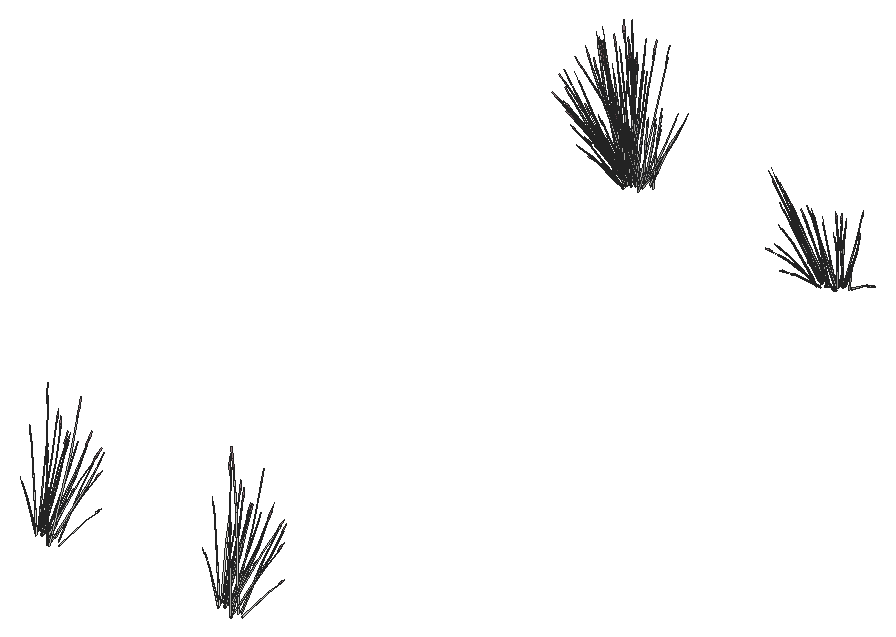
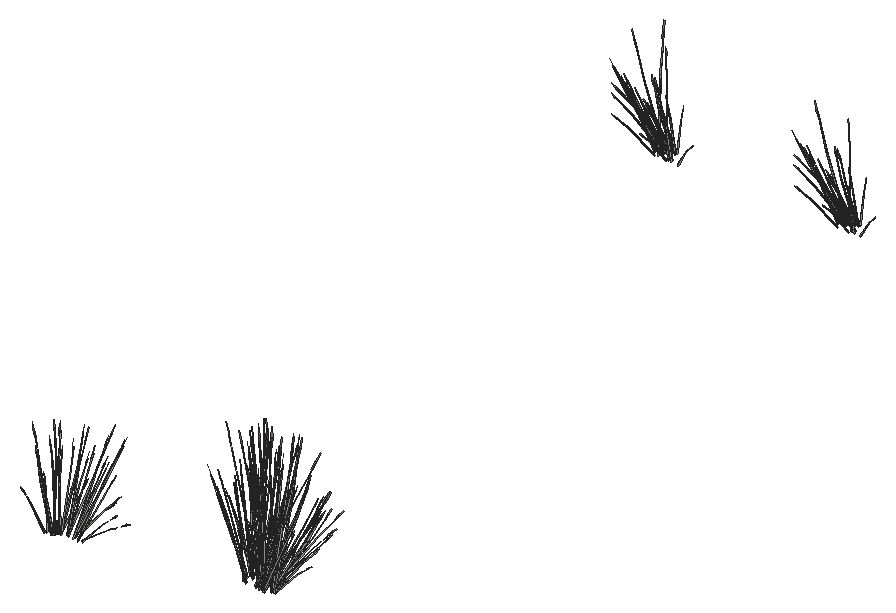
# SketchUp Ruby script. Lengths in millimetres.
U = 1.mm
M = Sketchup.active_model
def pt(a) = Geom::Point3d.new(a.map { |v| v * U })
def face(e, loops, mat)
  f = e.add_face(loops[0].map { |a| pt(a) })
  loops[1..].each { |l| e.add_face(l.map { |a| pt(a) }).erase! }
  f.material = f.back_material = mat if mat
  f
end
# faces: each face lists its corners as indices into pts; further lists are holes
def faces(e, pts, list, mat = nil) = list.each { |f| face(e, (f[0].is_a?(Array) ? f : [f]).map { |l| l.map { |i| pts[i] } }, mat) }
# xy, xz, yz: faces in a plane at the given z, y or x. An outline is a flat list of corners, or four numbers for a rectangle; further outlines are holes
def ring(l) = l.size == 4 ? [[l[0], l[1]], [l[2], l[1]], [l[2], l[3]], [l[0], l[3]]] : l.each_slice(2).to_a
def flat(e, list, mat, &to3) = list.each { |f| face(e, (f[0].is_a?(Array) ? f : [f]).map { |l| ring(l).map { |u, v| to3.(u, v) } }, mat) }
def xy(e, z, list, mat = nil) = flat(e, list, mat) { |x, y| [x, y, z] }
def xz(e, y, list, mat = nil) = flat(e, list, mat) { |x, z| [x, y, z] }
def yz(e, x, list, mat = nil) = flat(e, list, mat) { |y, z| [x, y, z] }
def lines(e, pts, list) = list.each { |a, b| e.add_line(pt(pts[a]), pt(pts[b])) }
# prism: a flat outline (further loops are holes) pulled along v
def prism(e, loops, v, mat = nil)
  f = face(e, loops, mat); d = Geom::Vector3d.new(v.map { |x| x * U })
  f.pushpull(f.normal.samedirection?(d) ? d.length : -d.length)
end
def box(e, o, s, mat = nil) = prism(e, [[o, [o[0] + s[0], o[1], o[2]], [o[0] + s[0], o[1] + s[1], o[2]], [o[0], o[1] + s[1], o[2]]]], [0, 0, s[2]], mat)
def at(x, y, z, deg = 0) = Geom::Transformation.translation(pt([x, y, z])) * Geom::Transformation.rotation(ORIGIN, Z_AXIS, deg.degrees)
def axes(o, x, y, z) = Geom::Transformation.new([*x, 0, *y, 0, *z, 0, *pt(o).to_a, 1])
def part(name) = M.definitions.add(name)
# library, detail: a bought-in or finely detailed component or shape, given as its bounding box
def library(name, o, s) = part(name).tap { |d| box(d.entities, o, s) }
def detail(e, o, s) = box(e.add_group.entities, o, s)
def put(e, d, t, mat = nil) = e.add_instance(d, t).tap { |i| i.material = mat if mat }
def group(e, t, mat = nil) = e.add_group.tap { |g| g.transformation = t; g.material = mat if mat }.entities
root = M.entities
M.materials.add("LightPink_Translucent").color = [144, 107, 117]
M.materials["LightPink_Translucent"].alpha = 0.8
c1 = part("blade")
p = [[54.7,5.3,558.8],[0,4.4,0],[2.3,11.5,0],[55.5,7.8,558.8],[58.2,7.8,558.8],[9.8,11.5,0],
  [62.9,5.7,838.2],[63,6,838.2],[63.4,6,838.2]]
faces(c1.entities,p,[[0,1,2,3],[4,5,2,3],[6,0,3,7],[7,3,4,8]])
c2 = part("seeds")
p = [[7.6,-2.7,35.1],[-0.2,-0.6,40.4],[-0.2,-0.8,0.9],[3.5,-1.8,-1.7],[7.5,-0.8,76.3],[3.7,0.2,78.9]]
faces(c2.entities,p,[[0,1,2,3],[1,0,4,5]],"LightPink_Translucent")
c3 = part("blade with seeds")
put(c3.entities,c1,at(0,0,0))
put(c3.entities,c2,axes([60.9,6.5,787.2],[1.5799,-0.05474,1.17369],[-0.12525,1.92788,0.29478],[-0.07173,-0.02425,1.56792]))
put(root,c3,axes([16276,4472.3,8464.8],[0.7662,1.03778,0],[-1.28187,0.57875,-0.51607],[-0.29196,0.13181,1.63711]))
put(root,c3,axes([14278.8,4481.2,8442.4],[0.08928,-0.14952,1.76342],[1.12407,-0.44035,-0.26939],[0.34078,0.22791,0.30037]))
put(root,c3,axes([16307,4481.2,8442.4],[0.08928,-0.14952,1.76342],[1.12407,-0.44035,-0.26939],[0.34078,0.22791,0.30037]))
put(root,c3,axes([14231.2,4367.9,8476.7],[-0.03348,-0.97511,1.41272],[1.51511,0.25277,0.59816],[-0.35835,0.53357,1.3335]))
put(root,c3,axes([16259.4,4367.9,8476.7],[-0.03348,-0.97511,1.41272],[1.51511,0.25277,0.59816],[-0.35835,0.53357,1.3335]))
put(root,c3,axes([14241.1,4394.9,8457.7],[0.44936,0.94823,-0.69212],[-1.29441,0.3415,-0.18165],[0.04967,0.32109,1.52773]))
put(root,c3,axes([16269.3,4394.9,8457.7],[0.44936,0.94823,-0.69212],[-1.29441,0.3415,-0.18165],[0.04967,0.32109,1.52773]))
put(root,c3,axes([14016.6,4477.9,8442.4],[0.16438,0.10347,1.76342],[0.27873,0.95868,-0.26939],[-0.36432,0.20444,0.30037]))
put(root,c3,axes([16044.8,4477.9,8442.4],[0.16438,0.10347,1.76342],[0.27873,0.95868,-0.26939],[-0.36432,0.20444,0.30037]))
put(root,c3,axes([14234.3,4463.5,8523.4],[1.20928,-0.24619,-0.51099],[0.21154,0.93233,-0.3958],[0.32481,0.26718,0.97773]))
put(root,c3,axes([16262.5,4463.5,8523.4],[1.20928,-0.24619,-0.51099],[0.21154,0.93233,-0.3958],[0.32481,0.26718,0.97773]))
put(root,c3,axes([14276.7,4487.5,8472.3],[-0.78586,-0.03248,1.0506],[0.51898,-0.68985,0.58006],[0.31045,0.24509,0.8241]))
put(root,c3,axes([16304.9,4487.5,8472.3],[-0.78586,-0.03248,1.0506],[0.51898,-0.68985,0.58006],[0.31045,0.24509,0.8241]))
put(root,c3,axes([14072.3,4412.9,8503],[0.22818,-0.35597,1.71376],[0.95725,0.73667,0.13857],[-0.43183,0.45914,0.73262]))
put(root,c3,axes([16100.5,4412.9,8503],[0.22818,-0.35597,1.71376],[0.95725,0.73667,0.13857],[-0.43183,0.45914,0.73262]))
put(root,c3,axes([14211.5,4445,8470.3],[0.02163,-0.34331,1.43002],[1.03345,-0.38348,-0.30754],[0.31903,0.4109,0.61141]))
put(root,c3,axes([16239.7,4445,8470.3],[0.02163,-0.34331,1.43002],[1.03345,-0.38348,-0.30754],[0.31903,0.4109,0.61141]))
put(root,c3,axes([14079.1,4463.9,8519.5],[-0.82919,0.54528,-0.35414],[-0.78493,-0.62262,0.4572],[-0.11943,0.31634,0.87481]))
put(root,c3,axes([16107.2,4463.9,8519.5],[-0.82919,0.54528,-0.35414],[-0.78493,-0.62262,0.4572],[-0.11943,0.31634,0.87481]))
put(root,c3,axes([14092.5,4517.7,8474.7],[-0.03171,-0.6158,1.1486],[0.7925,0.43922,0.84392],[-0.15586,0.29352,0.25299]))
put(root,c3,axes([16120.6,4517.7,8474.7],[-0.03171,-0.6158,1.1486],[0.7925,0.43922,0.84392],[-0.15586,0.29352,0.25299]))
put(root,c3,axes([14145.5,4480.3,8442.4],[0.19833,-0.05635,1.76342],[1.19302,0.31018,-0.26939],[0.03489,0.3496,0.30037]))
put(root,c3,axes([16173.6,4480.3,8442.4],[0.19833,-0.05635,1.76342],[1.19302,0.31018,-0.26939],[0.03489,0.3496,0.30037]))
put(root,c3,axes([14100,4457.3,8531.6],[0.87728,0.69587,-0.5672],[-0.92674,0.60943,-0.43934],[-0.13348,0.35356,1.08528]))
put(root,c3,axes([16128.2,4457.3,8531.6],[0.87728,0.69587,-0.5672],[-0.92674,0.60943,-0.43934],[-0.13348,0.35356,1.08528]))
put(root,c3,axes([14075.8,4483.9,8476.2],[1.11329,-0.1834,0.06507],[0.25594,0.73887,-0.86304],[-0.07058,0.37403,0.7736]))
put(root,c3,axes([16104,4483.9,8476.2],[1.11329,-0.1834,0.06507],[0.25594,0.73887,-0.86304],[-0.07058,0.37403,0.7736]))
put(root,c3,axes([14166.1,4474.5,8523.4],[1.20468,0.25962,-0.51099],[-0.41292,0.89013,-0.3958],[0.11046,0.35838,0.97773]))
put(root,c3,axes([16194.3,4474.5,8523.4],[1.20468,0.25962,-0.51099],[-0.41292,0.89013,-0.3958],[0.11046,0.35838,0.97773]))
put(root,c3,axes([14183.5,4427.8,8503],[-0.28013,-0.33252,1.71376],[1.29445,-0.27994,0.13857],[0.29256,0.52202,0.73262]))
put(root,c3,axes([16211.6,4427.8,8503],[-0.28013,-0.33252,1.71376],[1.29445,-0.27994,0.13857],[0.29256,0.52202,0.73262]))
put(root,c3,axes([14152.1,4488.3,8519.5],[-0.36946,0.79643,-0.35414],[-1.07787,-0.23229,0.4572],[0.09883,0.32066,0.87481]))
put(root,c3,axes([16180.3,4488.3,8519.5],[-0.36946,0.79643,-0.35414],[-1.07787,-0.23229,0.4572],[0.09883,0.32066,0.87481]))
put(root,c3,axes([14093.1,4449.3,8540.1],[-0.03189,0.95798,-0.7886],[-1.34277,-0.06434,0.09517],[-0.14171,0.40585,1.11556]))
put(root,c3,axes([16121.3,4449.3,8540.1],[-0.03189,0.95798,-0.7886],[-1.34277,-0.06434,0.09517],[-0.14171,0.40585,1.11556]))
put(root,c3,axes([14125.4,4432,8503],[-0.02999,-0.3975,1.71376],[1.30002,0.26369,0.13857],[-0.08041,0.56647,0.73262]))
put(root,c3,axes([16153.5,4432,8503],[-0.02999,-0.3975,1.71376],[1.30002,0.26369,0.13857],[-0.08041,0.56647,0.73262]))
put(root,c3,axes([14155,4470.2,8531],[0.5849,0.8421,-0.71045],[-1.20401,0.4693,0.08574],[0.13677,0.40688,1.00501]))
put(root,c3,axes([16183.1,4470.2,8531],[0.5849,0.8421,-0.71045],[-1.20401,0.4693,0.08574],[0.13677,0.40688,1.00501]))
put(root,c3,axes([14069,4503.8,8470.3],[0.38672,-0.16338,1.43002],[0.95481,0.49262,-0.30754],[-0.28419,0.42626,0.61141]))
put(root,c3,axes([16097.1,4503.8,8470.3],[0.38672,-0.16338,1.43002],[0.95481,0.49262,-0.30754],[-0.28419,0.42626,0.61141]))
put(root,c3,axes([14081.7,4483.5,8489.9],[0.02693,-0.53464,1.54345],[1.21102,0.2824,0.21329],[-0.10493,0.5698,0.72882]))
put(root,c3,axes([16109.8,4483.5,8489.9],[0.02693,-0.53464,1.54345],[1.21102,0.2824,0.21329],[-0.10493,0.5698,0.72882]))
put(root,c3,axes([14105.3,12509.6,8503],[0.28013,0.33252,1.71376],[-1.29445,0.27994,0.13857],[-0.29256,-0.52202,0.73262]))
put(root,c3,axes([14233.3,12497.3,8470.3],[-0.34835,0.20963,1.43002],[-1.04325,-0.36691,-0.30754],[0.19338,-0.4563,0.61141]))
put(root,c3,axes([14192.9,12515.9,8531],[-0.5849,-0.8421,-0.71045],[1.20401,-0.4693,0.08574],[-0.13677,-0.40688,1.00501]))
put(root,c3,axes([14096.3,12487.3,8470.3],[-0.07421,0.33879,1.43002],[-1.08488,0.28361,-0.30754],[-0.25359,-0.4379,0.61141]))
put(root,c3,axes([14167.3,12468.4,8442.4],[-0.20555,0.03731,1.76342],[-1.13672,-0.42002,-0.26939],[0.01907,-0.35034,0.30037]))
put(root,c3,axes([14254.8,12536.8,8531],[0.03189,-0.95798,-0.71045],[1.34277,0.06434,0.08574],[0.14171,-0.40585,1.00501]))
put(root,c3,axes([14195.8,12497.7,8519.5],[0.36946,-0.79643,-0.35414],[1.07787,0.23229,0.4572],[-0.09883,-0.32066,0.87481]))
put(root,c3,axes([14216.4,12524.4,8503],[-0.22818,0.35597,1.71376],[-0.95725,-0.73667,0.13857],[0.43183,-0.45914,0.73262]))
put(root,c3,axes([14181.8,12511.6,8523.4],[-1.20468,-0.25962,-0.51099],[0.41292,-0.89013,-0.3958],[-0.11046,-0.35838,0.97773]))
put(root,c3,axes([14200.7,12455,8474.7],[0.15721,0.60392,1.1486],[-0.87211,-0.33448,0.84392],[0.09385,-0.30923,0.25299]))
put(root,c3,axes([14247.9,12528.7,8523.4],[-0.87728,-0.69587,-0.51099],[0.92674,-0.60943,-0.3958],[0.13348,-0.35356,0.97773]))
put(root,c3,axes([16317.5,12508.8,8197],[-0.18744,-0.14521,1.74944],[-1.25089,0.09206,-0.27667],[-0.19964,-0.34731,0.14031]))
put(root,c3,axes([14268.9,12522.1,8519.5],[0.82919,-0.54528,-0.35414],[0.78493,0.62262,0.4572],[0.11943,-0.31634,0.87481]))
put(root,c3,axes([14086.8,12473.4,8474.7],[0.63926,0.36046,1.1486],[-0.93099,0.21668,0.84392],[-0.1992,-0.27702,0.25299]))
put(root,c3,axes([14126,12521.9,8531],[-1.04497,-0.50058,-0.71045],[0.74264,-0.8772,0.08574],[-0.3786,-0.29889,1.00501]))
put(root,c3,axes([14116.8,12505.1,8519.5],[-0.18927,-0.83419,-0.35414],[1.08199,-0.22027,0.4572],[-0.29062,-0.23905,0.87481]))
put(root,c3,axes([16460.2,12554,8197],[-0.01183,-0.20612,1.74944],[-0.99913,-0.59572,-0.27667],[0.15447,-0.36112,0.14031]))
put(root,c3,axes([16453.4,12535.2,8196.8],[-0.12446,0.07911,1.77383],[-1.21937,-0.26689,-0.16761],[-0.04414,-0.34521,0.31391]))
put(root,c3,axes([14074,12501,8442.4],[-0.11871,0.13643,1.76342],[-1.19964,0.29415,-0.26939],[-0.2898,-0.26759,0.30037]))
put(root,c3,axes([14124.2,12596.2,8457.8],[-0.50328,-1.06202,-0.69835],[1.44974,-0.38248,-0.18329],[-0.05563,-0.35963,1.54149]))
put(root,c3,axes([14057.7,12535.9,8503],[0.45521,0.17844,1.71376],[-0.94204,0.74856,0.13857],[-0.58713,-0.33769,0.73262]))
put(root,c3,axes([14295.1,12513.8,8442.4],[-0.18342,-0.08159,1.76342],[-0.47115,-0.9115,-0.26939],[0.31784,-0.24736,0.30037]))
put(root,c3,axes([16284.9,12496.7,8196.8],[-0.02286,0.12414,1.77383],[-1.12758,0.45052,-0.16761],[-0.33182,-0.23029,0.31391]))
put(root,c3,axes([14113.6,12522.6,8523.4],[-1.20928,0.24619,-0.51099],[-0.21154,-0.93233,-0.3958],[-0.32481,-0.26718,0.97773]))
put(root,c3,axes([16278.6,12552.6,8206.6],[1.36515,-0.26619,0.53763],[0.23692,1.04421,0.4433],[-0.32106,-0.30775,1.11249]))
put(root,c3,axes([16357,12557.6,8197.4],[1.20755,0.27075,0.48003],[-0.41292,0.89013,0.3958],[-0.07257,-0.35005,0.9933]))
put(root,c3,axes([16365.8,12565.7,8205.1],[-1.19922,0.48218,-0.1216],[-0.58932,-0.85579,-0.67495],[-0.15822,-0.36063,1.02557]))
put(root,c3,axes([16429.1,12593.2,8205.1],[-1.34686,-0.05131,-0.1216],[0.03681,-0.97156,-0.67495],[0.09356,-0.37418,1.02557]))
put(root,c3,axes([14295,12579.1,8531],[0.64013,-0.81717,-0.71045],[1.12174,0.58074,0.08574],[0.38221,-0.29607,1.00501]))
put(root,c3,axes([16365.1,12555.9,8197.4],[0.90301,-0.35198,0.0643],[0.44199,0.64184,0.50621],[-0.08721,-0.28293,0.77189]))
put(root,c3,axes([14119.2,12518.6,8464.8],[-0.7662,-1.03778,0],[1.28187,-0.57875,-0.51607],[0.29196,-0.13181,1.63711]))
put(root,c3,axes([14294.2,12569.4,8523.4],[-0.31482,-0.94565,-0.51099],[1.19224,-0.16542,-0.3958],[0.34166,-0.254,0.97773]))
put(root,c3,axes([14161.9,12486.9,8458.6],[-0.84686,0.59414,-0.03893],[-0.77596,-0.65071,-0.17649],[-0.05463,-0.18438,0.58215]))
put(root,c3,axes([16286.6,12558.4,8197.4],[0.55698,-0.6579,0.0643],[0.79316,0.38303,0.50621],[-0.25643,-0.21093,0.77189]))
put(root,c3,axes([14189.5,12665.8,8489],[1.05902,0.41762,1.51261],[-1.03748,0.89969,0.59816],[-0.46471,-0.53324,1.26806]))
put(root,c3,axes([14048.9,12592.4,8455.8],[0,-1.03566,-0.49651],[1.37109,0,0],[0,-0.23588,1.57504]))
put(root,c3,axes([14145.7,12514.6,8455.8],[1.14694,-0.51783,-0.49651],[0.68554,0.92854,0],[0.26122,-0.11794,1.57504]))
put(root,c3,axes([14318.5,12560,8470.3],[-0.4378,-0.03068,1.43002],[-0.44851,-0.8229,-0.30754],[0.53783,-0.23279,0.61141]))
put(root,c3,axes([14180.2,12568.5,8456.8],[0.82544,-0.77843,-0.62353],[1.0254,0.70586,-0.16365],[0.33076,-0.19418,1.37633]))
put(root,c3,axes([16356.6,12574.2,8205.5],[-0.36946,0.79643,0.35414],[-1.07787,-0.23229,-0.4572],[-0.09883,-0.32066,0.87481]))
put(root,c3,axes([14331.3,12521.6,8474.7],[-0.40819,0.5272,1.1486],[-0.35086,-0.70831,0.84392],[0.33713,-0.17749,0.25299]))
put(root,c3,axes([16426.6,12582.7,8197.4],[0.87265,0.70663,0.48003],[-0.92674,0.60943,0.3958],[0.16097,-0.33153,0.9933]))
put(root,c3,axes([16292.9,12556.6,8215.1],[-0.81789,0.99285,-0.13619],[-1.18445,-0.572,-0.75594],[-0.41173,-0.28051,1.14864]))
put(root,c3,axes([16434.8,12584.4,8197.4],[1.00708,0.04826,0.0643],[-0.02761,0.72867,0.50621],[0.10538,-0.27912,0.77189]))
put(root,c3,axes([14316.5,12571.9,8519.5],[1.06674,-0.14801,-0.35414],[0.28168,0.84611,0.4572],[0.30569,-0.22726,0.87481]))
put(root,c3,axes([16415.7,12597,8205.5],[-0.82919,0.54528,0.35414],[-0.78493,-0.62262,-0.4572],[0.11943,-0.31634,0.87481]))
put(root,c3,axes([14143.7,12603.2,8460.7],[0.59459,-0.93321,-0.44739],[1.23546,0.44912,0.21531],[0,-0.21512,1.43643]))
put(root,c3,axes([14053.2,12542.4,8519.5],[-0.69728,-0.64842,-0.35414],[0.79619,-0.61382,0.4572],[-0.40453,-0.09339,0.87481]))
put(root,c3,axes([14157.5,12591.4,8472.2],[-0.1428,-1.18174,-0.29095],[1.48733,-0.07145,-0.50002],[0.26191,-0.15741,1.59708]))
put(root,c3,axes([14063.8,12593,8456],[0.85545,-0.64616,-0.30978],[0.85545,0.64616,0.30978],[0,-0.20813,1.38974]))
put(root,c3,axes([14055,12514.3,8458.6],[-0.35352,0.84566,-0.03893],[-1.08806,-0.26014,-0.17649],[-0.1652,-0.13832,0.58215]))
put(root,c3,axes([14139.9,12622.9,8472.2],[-1.38012,-0.49416,-0.29095],[0.66454,-1.04299,-0.50002],[-0.04337,-0.25608,1.59708]))
put(root,c3,axes([16213.3,12549.4,8197],[-0.26368,-0.00731,1.74944],[-0.83946,0.73103,-0.27667],[-0.44791,-0.14937,0.14031]))
put(root,c3,axes([16466.3,12641.8,8205.1],[-1.1336,-0.57106,-0.1216],[0.65308,-0.827,-0.67495],[0.32027,-0.28747,1.02557]))
put(root,c3,axes([14040.2,12612.4,8464.8],[-1.53239,0,0],[0,-1.1575,-0.51607],[0,-0.26363,1.63711]))
put(root,c3,axes([14046.8,12559.9,8470.3],[0.23927,0.28834,1.43002],[-0.55135,0.78376,-0.30754],[-0.56612,-0.18733,0.61141]))
put(root,c3,axes([14152.5,12525,8456],[1.14332,0.25625,-0.30978],[-0.28787,0.90242,0.30978],[0.23049,-0.10406,1.38974]))
put(root,c3,axes([14071.9,12553.4,8531],[-1.22504,-0.02494,-0.71045],[0.08228,-1.05005,0.08574],[-0.51899,-0.11081,1.00501]))
put(root,c3,axes([16290.9,12577.6,8205.5],[0.18927,0.83419,0.35414],[-1.08199,0.22027,-0.4572],[-0.29062,-0.23905,0.87481]))
put(root,c3,axes([16208.4,12591.4,8206.6],[1.01205,-0.7643,0.53763],[0.87284,0.81167,0.4433],[-0.47482,-0.14098,1.11249]))
put(root,c3,axes([16537.2,12635.5,8196.8],[-0.16006,-0.00787,1.77383],[-0.66468,-0.8428,-0.16761],[0.26693,-0.27711,0.31391]))
put(root,c3,axes([14070.3,12604.6,8463.7],[-1.1399,0.87071,0.30756],[-1.1406,-0.86155,-0.36492],[-0.03981,-0.24727,1.64885]))
put(root,c3,axes([16220.1,12591.3,8197.4],[0.06171,-0.78753,0.0643],[0.9318,0.02159,0.50621],[-0.35694,-0.08241,0.77189]))
put(root,c3,axes([14162.4,12615,8466.3],[1.3808,0.50196,0.24065],[-0.66454,1.04299,0.50002],[0,-0.24043,1.60543]))
put(root,c3,axes([14148.7,12650.8,8466.5],[0.32481,-1.2272,-0.23429],[1.54007,0.21392,0.51271],[-0.26911,-0.16947,1.5644]))
put(root,c3,axes([14061.6,12558.8,8523.4],[-0.88986,0.68603,-0.51099],[-0.77932,-0.72471,-0.3958],[-0.45212,-0.10438,0.97773]))
put(root,c3,axes([16452.3,12639.8,8205.5],[-1.06674,0.14801,0.35414],[-0.28168,-0.84611,-0.4572],[0.30569,-0.22726,0.87481]))
put(root,c3,axes([14010.7,12581.8,8474.7],[0.78239,-0.07411,1.1486],[-0.49629,0.65296,0.84392],[-0.38663,-0.09795,0.25299]))
put(root,c3,axes([14151.1,12597.2,8473.6],[-1.33077,0.06393,0.44739],[-0.12035,-1.06125,-0.21531],[0.23824,-0.10756,1.43643]))
put(root,c3,axes([14063.8,12616.9,8467.5],[0,1.03566,0.49651],[-1.37109,0,0],[0,-0.23588,1.57504]))
put(root,c3,axes([14308.3,12622.7,8523.4],[0.332,-0.94205,-0.51099],[1.13828,0.3229,-0.3958],[0.45829,-0.08638,0.97773]))
put(root,c3,axes([14262.5,12525.3,8464.9],[0.7662,-1.03778,0],[1.28187,0.57875,-0.51607],[0.29196,0.13181,1.63711]))
put(root,c3,axes([14033.3,12577.4,8503],[0.50831,-0.02346,1.71376],[-0.33721,1.01661,0.13857],[-0.72439,-0.06288,0.73262]))
put(root,c3,axes([14146,12638.1,8460.7],[-0.73619,-0.86927,-0.44739],[1.11511,-0.61213,0.21531],[-0.23824,-0.10756,1.43643]))
put(root,c3,axes([14149.9,12606.9,8464.5],[0.53281,1.15808,0.45755],[-1.52239,0.4027,0.17955],[0.01861,-0.2128,1.58856]))
put(root,c3,axes([14339.1,12629.5,8454.9],[-0.7893,0.12429,1.41583],[-0.12563,-0.9893,0.08104],[0.55282,-0.14974,0.80566]))
put(root,c3,axes([14375.6,12607.2,8461.9],[-0.75977,-0.66224,-0.06488],[0.83212,-0.6068,-0.29416],[0.23578,-0.04272,0.97024]))
put(root,c3,axes([14143.1,12630.1,8473.6],[-0.59459,0.93321,0.44739],[-1.23546,-0.44912,-0.21531],[0,-0.21512,1.43643]))
put(root,c3,axes([16476.9,12636.4,8197.4],[0.8413,0.43556,0.0643],[-0.48981,0.62025,0.50621],[0.26973,-0.20053,0.77189]))
put(root,c3,axes([16470.9,12631.8,8197.4],[0.30393,0.95317,0.48003],[-1.19224,0.16542,0.3958],[0.35138,-0.22417,0.9933]))
put(root,c3,axes([14198.6,12609.4,8460.5],[0,-1.19833,0],[1.53239,0,0],[0,0,1.79456]))
put(root,c3,axes([16552.5,12661.1,8197],[0.17006,-0.15775,1.74944],[-0.21766,-0.96766,-0.27667],[0.42669,-0.18347,0.14031]))
put(root,c3,axes([14245.8,12539.1,8467.5],[-1.14694,-0.51783,0.49651],[0.68554,-0.92854,0],[0.26122,0.11794,1.57504]))
put(root,c3,axes([14302.8,12631.4,8531],[1.07686,-0.45739,-0.71045],[0.60013,0.94154,0.08574],[0.52031,-0.10696,1.00501]))
put(root,c3,axes([14129.2,12646.5,8456.8],[-1.27479,-0.1698,-0.62353],[0.26901,-1.04736,-0.16365],[-0.38043,-0.12691,1.37633]))
put(root,c3,axes([16187.5,12565.1,8196.8],[0.09085,0.10335,1.77383],[-0.43798,0.92907,-0.16761],[-0.44357,0.00672,0.31391]))
put(root,c3,axes([14180.1,12590.2,8464.5],[-1.01611,0.93987,0.45755],[-1.20717,-0.82966,0.17955],[0.24496,-0.0938,1.58856]))
put(root,c3,axes([14208.3,12633,8462.9],[-1.1399,-0.8914,-0.06131],[1.1406,-0.89194,0],[-0.03981,-0.03113,1.75571]))
